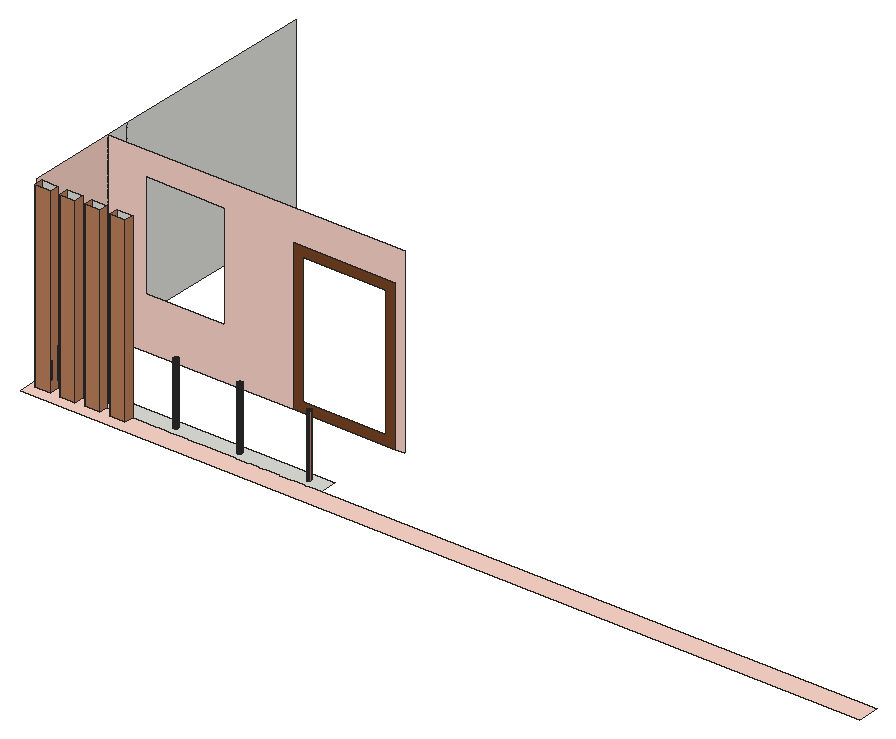
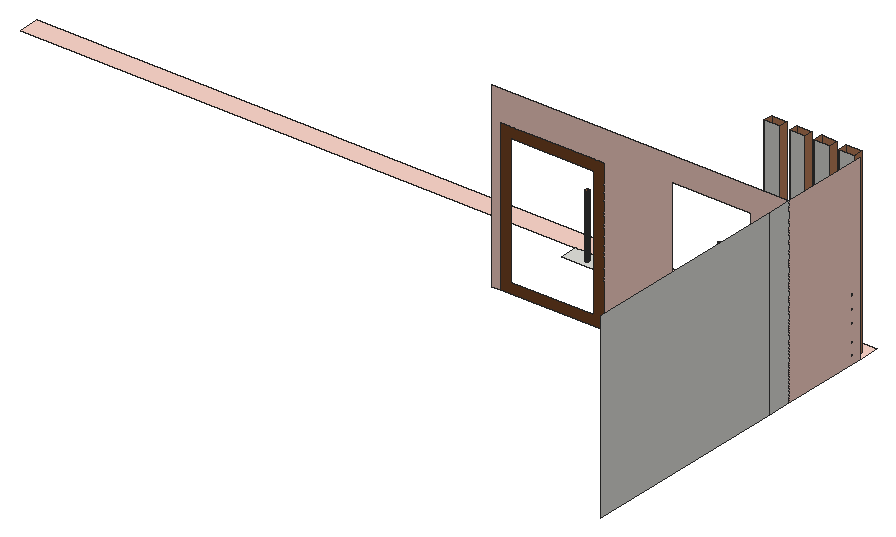
# SketchUp Ruby script. Lengths in inches.
U = 1.inch
M = Sketchup.active_model
def pt(a) = Geom::Point3d.new(a.map { |v| v * U })
def face(e, loops, mat)
  f = e.add_face(loops[0].map { |a| pt(a) })
  loops[1..].each { |l| e.add_face(l.map { |a| pt(a) }).erase! }
  f.material = f.back_material = mat if mat
  f
end
# faces: each face lists its corners as indices into pts; further lists are holes
def faces(e, pts, list, mat = nil) = list.each { |f| face(e, (f[0].is_a?(Array) ? f : [f]).map { |l| l.map { |i| pts[i] } }, mat) }
# xy, xz, yz: faces in a plane at the given z, y or x. An outline is a flat list of corners, or four numbers for a rectangle; further outlines are holes
def ring(l) = l.size == 4 ? [[l[0], l[1]], [l[2], l[1]], [l[2], l[3]], [l[0], l[3]]] : l.each_slice(2).to_a
def flat(e, list, mat, &to3) = list.each { |f| face(e, (f[0].is_a?(Array) ? f : [f]).map { |l| ring(l).map { |u, v| to3.(u, v) } }, mat) }
def xy(e, z, list, mat = nil) = flat(e, list, mat) { |x, y| [x, y, z] }
def xz(e, y, list, mat = nil) = flat(e, list, mat) { |x, z| [x, y, z] }
def yz(e, x, list, mat = nil) = flat(e, list, mat) { |y, z| [x, y, z] }
def lines(e, pts, list) = list.each { |a, b| e.add_line(pt(pts[a]), pt(pts[b])) }
# prism: a flat outline (further loops are holes) pulled along v
def prism(e, loops, v, mat = nil)
  f = face(e, loops, mat); d = Geom::Vector3d.new(v.map { |x| x * U })
  f.pushpull(f.normal.samedirection?(d) ? d.length : -d.length)
end
def box(e, o, s, mat = nil) = prism(e, [[o, [o[0] + s[0], o[1], o[2]], [o[0] + s[0], o[1] + s[1], o[2]], [o[0], o[1] + s[1], o[2]]]], [0, 0, s[2]], mat)
def at(x, y, z, deg = 0) = Geom::Transformation.translation(pt([x, y, z])) * Geom::Transformation.rotation(ORIGIN, Z_AXIS, deg.degrees)
def axes(o, x, y, z) = Geom::Transformation.new([*x, 0, *y, 0, *z, 0, *pt(o).to_a, 1])
def part(name) = M.definitions.add(name)
# library, detail: a bought-in or finely detailed component or shape, given as its bounding box
def library(name, o, s) = part(name).tap { |d| box(d.entities, o, s) }
def detail(e, o, s) = box(e.add_group.entities, o, s)
def put(e, d, t, mat = nil) = e.add_instance(d, t).tap { |i| i.material = mat if mat }
def group(e, t, mat = nil) = e.add_group.tap { |g| g.transformation = t; g.material = mat if mat }.entities
root = M.entities
M.materials.add("[Color B01]").color = [255, 216, 204]
M.materials.add("[Wood Veneer 01]1").color = [120, 70, 37]
M.materials.add("[Wood Veneer 02]").color = [190, 128, 91]
xy(root,1956.4375,[[[77.93,267.5625,1053.15,328.8],[114.33,291.11,112.32,291.37,110.45,292.15,108.85,293.38,107.62,294.98,106.84,296.85,106.58,298.86,106.84,300.86,107.62,302.73,108.85,304.34,110.45,305.57,112.32,306.34,114.33,306.61,116.34,306.34,118.2,305.57,119.81,304.34,121.04,302.73,121.82,300.86,122.08,298.86,121.82,296.85,121.04,294.98,119.81,293.38,118.2,292.15,116.34,291.37],[988.02,291.11,986.01,291.37,984.14,292.15,982.54,293.38,981.31,294.98,980.53,296.85,980.27,298.86,980.53,300.86,981.31,302.73,982.54,304.34,984.14,305.57,986.01,306.34,988.02,306.61,990.02,306.34,991.89,305.57,993.5,304.34,994.73,302.73,995.5,300.86,995.77,298.86,995.5,296.85,994.73,294.98,993.5,293.38,991.89,292.15,990.02,291.37],[309.08,291.11,307.07,291.37,305.2,292.15,303.6,293.38,302.37,294.98,301.59,296.85,301.33,298.86,301.59,300.86,302.37,302.73,303.6,304.34,305.2,305.57,307.07,306.34,309.08,306.61,311.09,306.34,312.95,305.57,314.56,304.34,315.79,302.73,316.57,300.86,316.83,298.86,316.57,296.85,315.79,294.98,314.56,293.38,312.95,292.15,311.09,291.37],[748.77,291.11,746.76,291.37,744.89,292.15,743.29,293.38,742.06,294.98,741.28,296.85,741.02,298.86,741.28,300.86,742.06,302.73,743.29,304.34,744.89,305.57,746.76,306.34,748.77,306.61,750.77,306.34,752.64,305.57,754.25,304.34,755.48,302.73,756.25,300.86,756.52,298.86,756.25,296.85,755.48,294.98,754.25,293.38,752.64,292.15,750.77,291.37],[530.58,291.11,528.57,291.37,526.7,292.15,525.1,293.38,523.87,294.98,523.09,296.85,522.83,298.86,523.09,300.86,523.87,302.73,525.1,304.34,526.7,305.57,528.57,306.34,530.58,306.61,532.59,306.34,534.45,305.57,536.06,304.34,537.29,302.73,538.07,300.86,538.33,298.86,538.07,296.85,537.29,294.98,536.06,293.38,534.45,292.15,532.59,291.37]],[114.33,291.11,112.32,291.37,110.45,292.15,108.85,293.38,107.62,294.98,106.84,296.85,106.58,298.86,106.84,300.86,107.62,302.73,108.85,304.34,110.45,305.57,112.32,306.34,114.33,306.61,116.34,306.34,118.2,305.57,119.81,304.34,121.04,302.73,121.82,300.86,122.08,298.86,121.82,296.85,121.04,294.98,119.81,293.38,118.2,292.15,116.34,291.37],[309.08,291.11,307.07,291.37,305.2,292.15,303.6,293.38,302.37,294.98,301.59,296.85,301.33,298.86,301.59,300.86,302.37,302.73,303.6,304.34,305.2,305.57,307.07,306.34,309.08,306.61,311.09,306.34,312.95,305.57,314.56,304.34,315.79,302.73,316.57,300.86,316.83,298.86,316.57,296.85,315.79,294.98,314.56,293.38,312.95,292.15,311.09,291.37],[530.58,291.11,528.57,291.37,526.7,292.15,525.1,293.38,523.87,294.98,523.09,296.85,522.83,298.86,523.09,300.86,523.87,302.73,525.1,304.34,526.7,305.57,528.57,306.34,530.58,306.61,532.59,306.34,534.45,305.57,536.06,304.34,537.29,302.73,538.07,300.86,538.33,298.86,538.07,296.85,537.29,294.98,536.06,293.38,534.45,292.15,532.59,291.37],[748.77,291.11,746.76,291.37,744.89,292.15,743.29,293.38,742.06,294.98,741.28,296.85,741.02,298.86,741.28,300.86,742.06,302.73,743.29,304.34,744.89,305.57,746.76,306.34,748.77,306.61,750.77,306.34,752.64,305.57,754.25,304.34,755.48,302.73,756.25,300.86,756.52,298.86,756.25,296.85,755.48,294.98,754.25,293.38,752.64,292.15,750.77,291.37],
  [988.02,291.11,986.01,291.37,984.14,292.15,982.54,293.38,981.31,294.98,980.53,296.85,980.27,298.86,980.53,300.86,981.31,302.73,982.54,304.34,984.14,305.57,986.01,306.34,988.02,306.61,990.02,306.34,991.89,305.57,993.5,304.34,994.73,302.73,995.5,300.86,995.77,298.86,995.5,296.85,994.73,294.98,993.5,293.38,991.89,292.15,990.02,291.37]])
xy(root,1956.4375,[[77.93,195.0625,2962.22,195.0625,2962.22,267.5625,405.93,267.5625,405.93,236.1875,352.87,236.1875,352.87,267.5625,318.62,267.5625,318.62,236.1875,265.56,236.1875,265.56,267.5625,233.75,267.5625,233.75,236.1875,180.68,236.1875,180.68,267.5625,148.18,267.5625,148.18,236.1875,95.12,236.1875,95.12,267.5625,77.93,267.5625]],"[Color B01]")
xz(root,236.1875,[[95.12,1956.4375,148.18,2577.9375],[180.68,1956.4375,233.75,2577.9375],[265.56,1956.4375,318.62,2577.9375],[352.87,1956.4375,405.93,2577.9375]],"[Wood Veneer 02]")
xz(root,267.5625,[[95.12,1956.4375,148.18,2577.9375],[180.68,1956.4375,233.75,2577.9375],[265.56,1956.4375,318.62,2577.9375],[352.87,1956.4375,405.93,2577.9375]])
xz(root,571.9,[[[77.93,1956.4375,713.53,1956.4375,713.53,2470.75,1067.28,2470.75,1067.28,1956.4375,1096.47,1956.4375,1096.47,2577.9375,77.93,2577.9375],[206.78,2135.23,480.91,2496.04]]],"[Color B01]")
xz(root,571.9,[[[713.53,1956.4375,1067.28,2470.75],[747.7,1990.6,1033.12,2436.59]]],"[Wood Veneer 01]1")
yz(root,77.93,[[571.9,1956.4375,653.97,2577.9375],[653.97,1956.4375,1377.24,2577.9375]])
yz(root,77.93,[[[267.5625,1956.4375,571.9,2577.9375],[300.84,2017.49,299.33,2017.69,297.93,2018.27,296.73,2019.2,295.8,2020.4,295.22,2021.8,295.02,2023.31,295.22,2024.8125,295.8,2026.21,296.73,2027.42,297.93,2028.34,299.33,2028.92,300.84,2029.12,302.34,2028.92,303.74,2028.34,304.95,2027.42,305.87,2026.21,306.45,2024.8125,306.65,2023.31,306.45,2021.8,305.87,2020.4,304.95,2019.2,303.74,2018.27,302.34,2017.69],[300.84,1977.93,299.33,1978.13,297.93,1978.71,296.73,1979.63,295.8,1980.84,295.22,1982.24,295.02,1983.74,295.22,1985.25,295.8,1986.65,296.73,1987.85,297.93,1988.78,299.33,1989.36,300.84,1989.56,302.34,1989.36,303.74,1988.78,304.95,1987.85,305.87,1986.65,306.45,1985.25,306.65,1983.74,306.45,1982.24,305.87,1980.84,304.95,1979.63,303.74,1978.71,302.34,1978.13],[300.84,2076.99,299.33,2077.19,297.93,2077.77,296.73,2078.7,295.8,2079.9,295.22,2081.3,295.02,2082.81,295.22,2084.3125,295.8,2085.71,296.73,2086.92,297.93,2087.84,299.33,2088.42,300.84,2088.62,302.34,2088.42,303.74,2087.84,304.95,2086.92,305.87,2085.71,306.45,2084.3125,306.65,2082.81,306.45,2081.3,305.87,2079.9,304.95,2078.7,303.74,2077.77,302.34,2077.19],[300.84,2119.12,299.33,2119.32,297.93,2119.9,296.73,2120.82,295.8,2122.03,295.22,2123.43,295.02,2124.93,295.22,2126.4375,295.8,2127.84,296.73,2129.04,297.93,2129.97,299.33,2130.55,300.84,2130.74,302.34,2130.55,303.74,2129.97,304.95,2129.04,305.87,2127.84,306.45,2126.4375,306.65,2124.93,306.45,2123.43,305.87,2122.03,304.95,2120.82,303.74,2119.9,302.34,2119.32],[300.84,2164.31,299.33,2164.51,297.93,2165.09,296.73,2166.01,295.8,2167.21,295.22,2168.62,295.02,2170.12,295.22,2171.625,295.8,2173.03,296.73,2174.23,297.93,2175.15,299.33,2175.73,300.84,2175.93,302.34,2175.73,303.74,2175.15,304.95,2174.23,305.87,2173.03,306.45,2171.625,306.65,2170.12,306.45,2168.62,305.87,2167.21,304.95,2166.01,303.74,2165.09,302.34,2164.51]]],"[Color B01]")
yz(root,95.12,[[236.1875,1956.4375,267.5625,2577.9375]],"[Wood Veneer 02]")
yz(root,148.18,[[236.1875,1956.4375,267.5625,2577.9375]],"[Wood Veneer 02]")
yz(root,180.68,[[236.1875,1956.4375,267.5625,2577.9375]],"[Wood Veneer 02]")
yz(root,233.75,[[236.1875,1956.4375,267.5625,2577.9375]],"[Wood Veneer 02]")
yz(root,265.56,[[236.1875,1956.4375,267.5625,2577.9375]],"[Wood Veneer 02]")
yz(root,318.62,[[236.1875,1956.4375,267.5625,2577.9375]],"[Wood Veneer 02]")
yz(root,352.87,[[236.1875,1956.4375,267.5625,2577.9375]],"[Wood Veneer 02]")
yz(root,405.93,[[236.1875,1956.4375,267.5625,2577.9375]],"[Wood Veneer 02]")
p = [[112.32,291.37,1956.4375],[114.33,291.11,1956.4375],[114.33,291.11,2172.125],[112.32,291.37,2172.125],[116.34,291.37,1956.4375],[116.34,291.37,2172.125],
  [307.07,291.37,1956.4375],[309.08,291.11,1956.4375],[309.08,291.11,2173.03],[307.07,291.37,2173.03],[311.09,291.37,1956.4375],[311.09,291.37,2173.03],
  [528.57,291.37,1956.4375],[530.58,291.11,1956.4375],[530.58,291.11,2169.25],[528.57,291.37,2169.25],[532.59,291.37,1956.4375],[532.59,291.37,2169.25],
  [746.76,291.37,1956.4375],[748.77,291.11,1956.4375],[748.77,291.11,2170.6875],[746.76,291.37,2170.6875],[750.77,291.37,1956.4375],[750.77,291.37,2170.6875],
  [986.01,291.37,1956.4375],[988.02,291.11,1956.4375],[988.02,291.11,2170.12],[986.01,291.37,2170.12],[990.02,291.37,1956.4375],[990.02,291.37,2170.12],
  [110.45,292.15,1956.4375],[110.45,292.15,2172.125],[118.2,292.15,1956.4375],[118.2,292.15,2172.125],[305.2,292.15,1956.4375],[305.2,292.15,2173.03],
  [312.95,292.15,1956.4375],[312.95,292.15,2173.03],[526.7,292.15,1956.4375],[526.7,292.15,2169.25],[534.45,292.15,1956.4375],[534.45,292.15,2169.25],
  [744.89,292.15,1956.4375],[744.89,292.15,2170.6875],[752.64,292.15,1956.4375],[752.64,292.15,2170.6875],[984.14,292.15,1956.4375],[984.14,292.15,2170.12],
  [991.89,292.15,1956.4375],[991.89,292.15,2170.12],[108.85,293.38,1956.4375],[108.85,293.38,2172.125],[119.81,293.38,1956.4375],[119.81,293.38,2172.125],
  [303.6,293.38,1956.4375],[303.6,293.38,2173.03],[314.56,293.38,1956.4375],[314.56,293.38,2173.03],[525.1,293.38,1956.4375],[525.1,293.38,2169.25],
  [536.06,293.38,1956.4375],[536.06,293.38,2169.25],[743.29,293.38,1956.4375],[743.29,293.38,2170.6875],[754.25,293.38,1956.4375],[754.25,293.38,2170.6875],
  [982.54,293.38,1956.4375],[982.54,293.38,2170.12],[993.5,293.38,1956.4375],[993.5,293.38,2170.12],[107.62,294.98,1956.4375],[107.62,294.98,2172.125],
  [121.04,294.98,1956.4375],[121.04,294.98,2172.125],[302.37,294.98,1956.4375],[302.37,294.98,2173.03],[315.79,294.98,1956.4375],[315.79,294.98,2173.03],
  [523.87,294.98,1956.4375],[523.87,294.98,2169.25],[537.29,294.98,1956.4375],[537.29,294.98,2169.25],[742.06,294.98,1956.4375],[742.06,294.98,2170.6875],
  [755.48,294.98,1956.4375],[755.48,294.98,2170.6875],[981.31,294.98,1956.4375],[981.31,294.98,2170.12],[994.73,294.98,1956.4375],[994.73,294.98,2170.12],
  [106.84,296.85,1956.4375],[106.84,296.85,2172.125],[121.82,296.85,1956.4375],[121.82,296.85,2172.125],[301.59,296.85,1956.4375],[302.03,295.8,2173.03],
  [301.59,296.85,2173.03],[316.57,296.85,1956.4375],[316.57,296.85,2173.03],[316.13,295.8,2173.03],[523.09,296.85,1956.4375],[523.09,296.85,2169.25],
  [538.07,296.85,1956.4375],[538.07,296.85,2169.25],[741.28,296.85,1956.4375],[741.28,296.85,2170.6875],[756.25,296.85,1956.4375],[756.25,296.85,2170.6875],
  [980.53,296.85,1956.4375],[981.29,295.02,2170.12],[980.53,296.85,2170.12],[995.5,296.85,1956.4375],[995.5,296.85,2170.12],[994.75,295.02,2170.12],
  [106.58,298.86,1956.4375],[106.58,298.86,2172.125],[122.08,298.86,1956.4375],[122.08,298.86,2172.125],[301.33,298.86,1956.4375],[301.33,298.86,2173.03],
  [316.83,298.86,1956.4375],[316.83,298.86,2173.03],[522.83,298.86,1956.4375],[522.83,298.86,2169.25],[538.33,298.86,1956.4375],[538.33,298.86,2169.25],
  [741.02,298.86,1956.4375],[741.02,298.86,2170.6875],[756.52,298.86,1956.4375],[756.52,298.86,2170.6875],[980.27,298.86,1956.4375],[980.27,298.86,2170.12],
  [106.84,300.86,1956.4375],[106.84,300.86,2172.125],[121.82,300.86,1956.4375],[121.82,300.86,2172.125],[301.59,300.86,1956.4375],[301.59,300.86,2173.03],
  [316.57,300.86,1956.4375],[316.57,300.86,2173.03],[523.09,300.86,1956.4375],[523.09,300.86,2169.25],[538.07,300.86,1956.4375],[538.07,300.86,2169.25],
  [741.28,300.86,1956.4375],[741.28,300.86,2170.6875],[756.25,300.86,1956.4375],[756.25,300.86,2170.6875],[980.53,300.86,1956.4375],[980.53,300.86,2170.12],
  [107.62,302.73,1956.4375],[107.62,302.73,2172.125],[121.04,302.73,1956.4375],[121.04,302.73,2172.125],[302.37,302.73,1956.4375],[302.37,302.73,2173.03],
  [315.79,302.73,1956.4375],[315.79,302.73,2173.03],[523.87,302.73,1956.4375],[523.87,302.73,2169.25],[537.29,302.73,1956.4375],[537.29,302.73,2169.25],
  [742.06,302.73,1956.4375],[742.06,302.73,2170.6875],[755.48,302.73,1956.4375],[755.48,302.73,2170.6875],[981.31,302.73,1956.4375],[981.31,302.73,2170.12],
  [995.5,300.86,1956.4375],[994.73,302.73,1956.4375],[994.73,302.73,2170.12],[995.5,300.86,2170.12],[108.85,304.34,1956.4375],[108.85,304.34,2172.125],
  [119.81,304.34,1956.4375],[119.81,304.34,2172.125],[303.6,304.34,1956.4375],[303.6,304.34,2173.03],[314.56,304.34,1956.4375],[314.56,304.34,2173.03],
  [525.1,304.34,1956.4375],[525.1,304.34,2169.25],[536.06,304.34,1956.4375],[536.06,304.34,2169.25],[743.29,304.34,1956.4375],[743.29,304.34,2170.6875],
  [754.25,304.34,1956.4375],[754.25,304.34,2170.6875],[982.54,304.34,1956.4375],[982.54,304.34,2170.12],[993.5,304.34,1956.4375],[993.5,304.34,2170.12],
  [110.45,305.57,1956.4375],[110.45,305.57,2172.125],[118.2,305.57,1956.4375],[118.2,305.57,2172.125],[305.2,305.57,1956.4375],[305.2,305.57,2173.03],
  [312.95,305.57,1956.4375],[312.95,305.57,2173.03],[526.7,305.57,1956.4375],[526.7,305.57,2169.25],[534.45,305.57,1956.4375],[534.45,305.57,2169.25],
  [744.89,305.57,1956.4375],[744.89,305.57,2170.6875],[752.64,305.57,1956.4375],[752.64,305.57,2170.6875],[984.14,305.57,1956.4375],[984.14,305.57,2170.12],
  [991.89,305.57,1956.4375],[991.89,305.57,2170.12],[112.32,306.34,1956.4375],[112.32,306.34,2172.125],[116.34,306.34,1956.4375],[116.34,306.34,2172.125],
  [307.07,306.34,1956.4375],[305.93,305.87,2173.03],[307.07,306.34,2173.03],[311.09,306.34,1956.4375],[311.09,306.34,2173.03],[312.23,305.87,2173.03],
  [528.57,306.34,1956.4375],[528.57,306.34,2169.25],[532.59,306.34,1956.4375],[532.59,306.34,2169.25],[746.76,306.34,1956.4375],[746.76,306.34,2170.6875],
  [750.77,306.34,1956.4375],[750.77,306.34,2170.6875],[986.01,306.34,1956.4375],[986.01,306.34,2170.12],[990.02,306.34,1956.4375],[990.02,306.34,2170.12],
  [114.33,306.61,1956.4375],[114.33,306.61,2172.125],[309.08,306.61,1956.4375],[309.08,306.61,2173.03],[530.58,306.61,1956.4375],[530.58,306.61,2169.25],
  [748.77,306.61,1956.4375],[748.77,306.61,2170.6875],[988.02,306.61,1956.4375],[988.02,306.61,2170.12]]
faces(root,p,[[0,1,2,3],[1,4,5,2],[30,0,3,31],[4,32,33,5],[50,30,31,51],[32,52,53,33],[70,50,51,71],[52,72,73,53],
  [90,70,71,91],[72,92,93,73],[114,90,91,115],[92,116,117,93],[132,114,115,133],[116,134,135,117],[150,132,133,151],[134,152,153,135],
  [172,150,151,173],[152,174,175,153],[192,172,173,193],[174,194,195,175],[212,192,193,213],[194,214,215,195],[234,212,213,235],[214,234,235,215]])
faces(root,p,[[6,7,8,9],[7,10,11,8],[12,13,14,15],[13,16,17,14],[18,19,20,21],[19,22,23,20],[24,25,26,27],[25,28,29,26],
  [34,6,9,35],[10,36,37,11],[38,12,15,39],[16,40,41,17],[42,18,21,43],[22,44,45,23],[46,24,27,47],[28,48,49,29],
  [54,34,35,55],[36,56,57,37],[58,38,39,59],[40,60,61,41],[62,42,43,63],[44,64,65,45],[66,46,47,67],[48,68,69,49],
  [74,54,55,75],[56,76,77,57],[78,58,59,79],[60,80,81,61],[82,62,63,83],[64,84,85,65],[86,66,67,87],[68,88,89,69],
  [94,74,75,95,96],[76,97,98,99,77],[100,78,79,101],[80,102,103,81],[104,82,83,105],[84,106,107,85],[108,86,87,109,110],[88,111,112,113,89],
  [118,94,96,119],[97,120,121,98],[122,100,101,123],[102,124,125,103],[126,104,105,127],[106,128,129,107],[130,108,110,131],[136,118,119,137],
  [120,138,139,121],[140,122,123,141],[124,142,143,125],[144,126,127,145],[128,146,147,129],[148,130,131,149],[154,136,137,155],[138,156,157,139],
  [158,140,141,159],[142,160,161,143],[162,144,145,163],[146,164,165,147],[166,148,149,167],[168,169,170,171],[176,154,155,177],[156,178,179,157],
  [180,158,159,181],[160,182,183,161],[184,162,163,185],[164,186,187,165],[188,166,167,189],[169,190,191,170],[196,176,177,197],[178,198,199,179],
  [200,180,181,201],[182,202,203,183],[204,184,185,205],[186,206,207,187],[208,188,189,209],[190,210,211,191],[216,196,197,217,218],[198,219,220,221,199],
  [222,200,201,223],[202,224,225,203],[226,204,205,227],[206,228,229,207],[230,208,209,231],[210,232,233,211],[236,216,218,237],[219,236,237,220],
  [238,222,223,239],[224,238,239,225],[240,226,227,241],[228,240,241,229],[242,230,231,243],[232,242,243,233]],"[Wood Veneer 02]")
